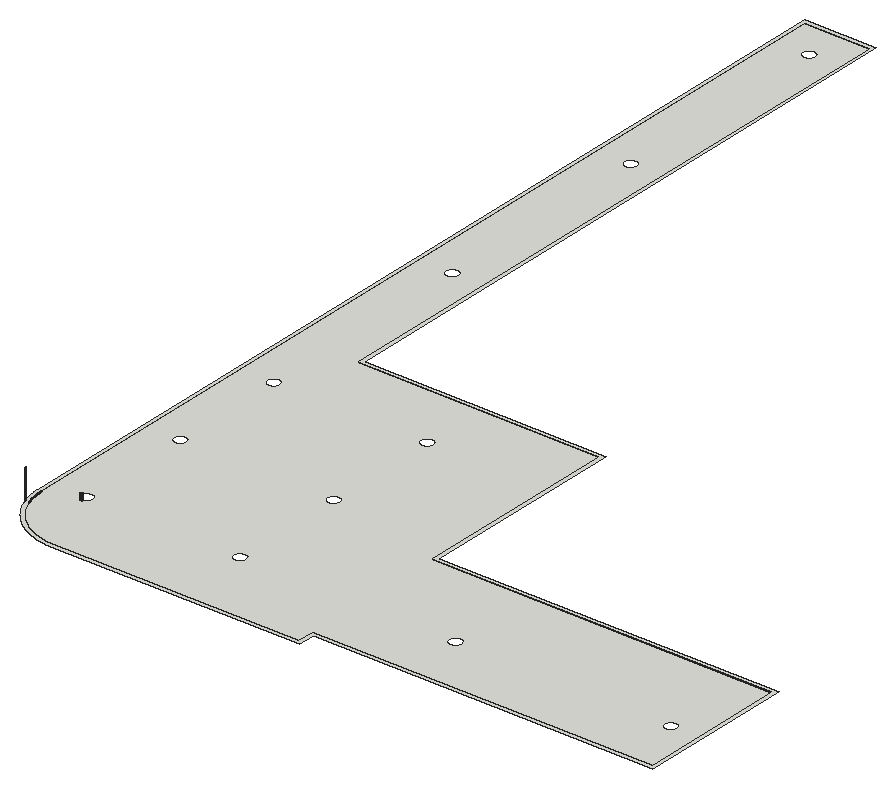
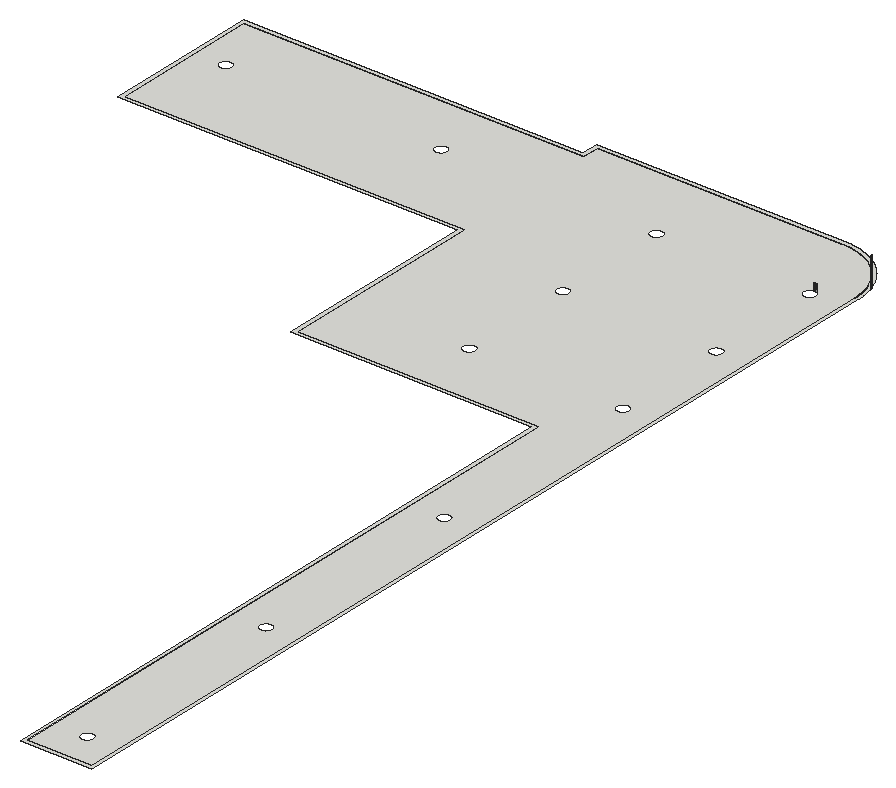
# SketchUp Ruby script. Lengths in inches.
U = 1.inch
M = Sketchup.active_model
def pt(a) = Geom::Point3d.new(a.map { |v| v * U })
def face(e, loops, mat)
  f = e.add_face(loops[0].map { |a| pt(a) })
  loops[1..].each { |l| e.add_face(l.map { |a| pt(a) }).erase! }
  f.material = f.back_material = mat if mat
  f
end
# faces: each face lists its corners as indices into pts; further lists are holes
def faces(e, pts, list, mat = nil) = list.each { |f| face(e, (f[0].is_a?(Array) ? f : [f]).map { |l| l.map { |i| pts[i] } }, mat) }
# xy, xz, yz: faces in a plane at the given z, y or x. An outline is a flat list of corners, or four numbers for a rectangle; further outlines are holes
def ring(l) = l.size == 4 ? [[l[0], l[1]], [l[2], l[1]], [l[2], l[3]], [l[0], l[3]]] : l.each_slice(2).to_a
def flat(e, list, mat, &to3) = list.each { |f| face(e, (f[0].is_a?(Array) ? f : [f]).map { |l| ring(l).map { |u, v| to3.(u, v) } }, mat) }
def xy(e, z, list, mat = nil) = flat(e, list, mat) { |x, y| [x, y, z] }
def xz(e, y, list, mat = nil) = flat(e, list, mat) { |x, z| [x, y, z] }
def yz(e, x, list, mat = nil) = flat(e, list, mat) { |y, z| [x, y, z] }
def lines(e, pts, list) = list.each { |a, b| e.add_line(pt(pts[a]), pt(pts[b])) }
# prism: a flat outline (further loops are holes) pulled along v
def prism(e, loops, v, mat = nil)
  f = face(e, loops, mat); d = Geom::Vector3d.new(v.map { |x| x * U })
  f.pushpull(f.normal.samedirection?(d) ? d.length : -d.length)
end
def box(e, o, s, mat = nil) = prism(e, [[o, [o[0] + s[0], o[1], o[2]], [o[0] + s[0], o[1] + s[1], o[2]], [o[0], o[1] + s[1], o[2]]]], [0, 0, s[2]], mat)
def at(x, y, z, deg = 0) = Geom::Transformation.translation(pt([x, y, z])) * Geom::Transformation.rotation(ORIGIN, Z_AXIS, deg.degrees)
def axes(o, x, y, z) = Geom::Transformation.new([*x, 0, *y, 0, *z, 0, *pt(o).to_a, 1])
def part(name) = M.definitions.add(name)
# library, detail: a bought-in or finely detailed component or shape, given as its bounding box
def library(name, o, s) = part(name).tap { |d| box(d.entities, o, s) }
def detail(e, o, s) = box(e.add_group.entities, o, s)
def put(e, d, t, mat = nil) = e.add_instance(d, t).tap { |i| i.material = mat if mat }
def group(e, t, mat = nil) = e.add_group.tap { |g| g.transformation = t; g.material = mat if mat }.entities
root = M.entities
M.materials.add("1496 AP 8293 CARBON COPY").color = [58, 58, 58]
xy(root,129,[[[43.625,86.5,43.25,86.51,42.88,86.52,42.51,86.54,42.14,86.5625,41.76,86.59,41.39,86.62,40.28,86.74,39.91,86.79,39.17,86.91,38.81,86.98,38.07,87.12,37.71,87.2,37.35,87.29,36.98,87.375,36.625,87.47,36.26,87.57,35.91,87.67,35.19,87.89,34.49,88.13,33.79,88.39,33.4375,88.53,33.09,88.67,32.75,88.8125,32.41,88.96,31.73,89.28,31.39,89.4375,31.0625,89.61,30.73,89.78,30.4,89.95,30.07,90.13,29.11,90.7,28.79,90.9,28.17,91.3,27.86,91.51,27.55,91.73,27.25,91.94,26.95,92.16,26.65,92.39,26.36,92.62,26.0625,92.85,25.78,93.09,25.49,93.33,25.21,93.57,24.65,94.07,24.11,94.59,23.59,95.11,23.07,95.65,22.57,96.21,22.33,96.49,22.09,96.78,21.85,97.0625,21.62,97.36,21.39,97.65,21.16,97.95,20.94,98.25,20.73,98.55,20.51,98.86,20.3,99.17,19.9,99.79,19.7,100.11,19.13,101.07,18.95,101.4,18.78,101.73,18.61,102.0625,18.4375,102.39,18.28,102.73,17.96,103.41,17.8125,103.75,17.67,104.09,17.53,104.4375,17.39,104.79,17.13,105.49,16.89,106.19,16.67,106.91,16.57,107.26,16.47,107.625,16.375,107.98,16.29,108.35,16.2,108.71,16.12,109.07,15.98,109.81,15.91,110.17,15.79,110.91,15.74,111.28,15.62,112.39,15.59,112.76,15.5625,113.14,15.54,113.51,15.52,113.88,15.51,114.25,15.5,114.625,15.5,553.5,45.5,553.5,45.5,259.5,156.5,259.5,156.5,163.5,312.5,163.5,312.5,94.5,156.5,94.5,156.5,86.5],[30.34,534,30.66,534,30.74,534.01,30.8125,534.02,30.89,534.03,31.05,534.05,31.125,534.07,31.2,534.08,31.28,534.1,31.35,534.125,31.43,534.15,31.5,534.17,31.58,534.2,31.79,534.29,31.86,534.33,31.93,534.36,32.07,534.44,32.13,534.48,32.2,534.53,32.26,534.57,32.33,534.62,32.57,534.82,32.62,534.88,32.68,534.93,32.88,535.17,32.93,535.24,32.97,535.3,33.02,535.37,33.06,535.43,33.14,535.57,33.17,535.64,33.21,535.71,33.3,535.92,33.33,536,33.35,536.07,33.375,536.15,33.4,536.22,33.42,536.3,33.43,536.375,33.45,536.45,33.47,536.61,33.48,536.6875,33.49,536.76,33.5,536.84,33.5,537.16,33.49,537.24,33.48,537.3125,33.47,537.39,33.45,537.55,33.43,537.625,33.42,537.7,33.4,537.78,33.375,537.85,33.35,537.93,33.33,538,33.3,538.08,33.21,538.29,33.17,538.36,33.14,538.43,33.06,538.57,33.02,538.63,32.97,538.7,32.93,538.76,32.88,538.83,32.68,539.07,32.62,539.12,32.57,539.18,32.33,539.38,32.26,539.43,32.2,539.47,32.13,539.52,32.07,539.56,31.93,539.64,31.86,539.67,31.79,539.71,31.58,539.8,31.5,539.83,31.43,539.85,31.35,539.875,31.28,539.9,31.2,539.92,31.125,539.93,31.05,539.95,30.89,539.97,30.8125,539.98,30.74,539.99,30.66,540,30.34,540,30.26,539.99,30.1875,539.98,30.11,539.97,29.95,539.95,29.875,539.93,29.8,539.92,29.72,539.9,29.65,539.875,29.57,539.85,29.5,539.83,29.42,539.8,29.21,539.71,29.14,539.67,29.07,539.64,28.93,539.56,28.87,539.52,28.8,539.47,28.74,539.43,28.67,539.38,28.43,539.18,28.38,539.12,28.32,539.07,28.12,538.83,28.07,538.76,28.03,538.7,27.98,538.63,27.94,538.57,27.86,538.43,27.83,538.36,27.79,538.29,27.7,538.08,27.67,538,27.65,537.93,27.625,537.85,27.6,537.78,27.58,537.7,27.57,537.625,27.55,537.55,27.53,537.39,27.52,537.3125,27.51,537.24,27.5,537.16,27.5,536.84,27.51,536.76,27.52,536.6875,27.53,536.61,27.55,536.45,27.57,536.375,27.58,536.3,27.6,536.22,27.625,536.15,27.65,536.07,27.67,536,27.7,535.92,27.79,535.71,27.83,535.64,27.86,535.57,27.94,535.43,27.98,535.37,28.03,535.3,28.07,535.24,28.12,535.17,28.32,534.93,28.38,534.88,28.43,534.82,28.67,534.62,28.74,534.57,28.8,534.53,28.87,534.48,28.93,534.44,29.07,534.36,29.14,534.33,29.21,534.29,29.42,534.2,29.5,534.17,29.57,534.15,29.65,534.125,29.72,534.1,29.8,534.08,29.875,534.07,29.95,534.05,30.11,534.03,30.1875,534.02,30.26,534.01],[30.34,329,30.66,329,30.74,329.01,30.8125,329.02,30.89,329.03,31.05,329.05,31.125,329.07,31.2,329.08,31.28,329.1,31.35,329.125,31.43,329.15,31.5,329.17,31.58,329.2,31.79,329.29,31.86,329.33,31.93,329.36,32.07,329.44,32.13,329.48,32.2,329.53,32.26,329.57,32.33,329.62,32.57,329.82,32.62,329.88,32.68,329.93,32.88,330.17,32.93,330.24,32.97,330.3,33.02,330.37,33.06,330.43,33.14,330.57,33.17,330.64,33.21,330.71,33.3,330.92,33.33,331,33.35,331.07,33.375,331.15,33.4,331.22,33.42,331.3,33.43,331.375,33.45,331.45,33.47,331.61,33.48,331.6875,33.49,331.76,33.5,331.84,33.5,332.16,33.49,332.24,33.48,332.3125,33.47,332.39,33.45,332.55,33.43,332.625,33.42,332.7,33.4,332.78,33.375,332.85,33.35,332.93,33.33,333,33.3,333.08,33.21,333.29,33.17,333.36,33.14,333.43,33.06,333.57,33.02,333.63,32.97,333.7,32.93,333.76,32.88,333.83,32.68,334.07,32.62,334.12,32.57,334.18,32.33,334.38,32.26,334.43,32.2,334.47,32.13,334.52,32.07,334.56,31.93,334.64,31.86,334.67,31.79,334.71,31.58,334.8,31.5,334.83,31.43,334.85,31.35,334.875,31.28,334.9,31.2,334.92,31.125,334.93,31.05,334.95,30.89,334.97,30.8125,334.98,30.74,334.99,30.66,335,30.34,335,30.26,334.99,30.1875,334.98,30.11,334.97,29.95,334.95,29.875,334.93,29.8,334.92,29.72,334.9,29.65,334.875,29.57,334.85,29.5,334.83,29.42,334.8,29.21,334.71,29.14,334.67,29.07,334.64,28.93,334.56,28.87,334.52,28.8,334.47,28.74,334.43,28.67,334.38,28.43,334.18,28.38,334.12,28.32,334.07,28.12,333.83,28.07,333.76,28.03,333.7,27.98,333.63,27.94,333.57,27.86,333.43,27.83,333.36,27.79,333.29,27.7,333.08,27.67,333,27.65,332.93,27.625,332.85,27.6,332.78,27.58,332.7,27.57,332.625,27.55,332.55,27.53,332.39,27.52,332.3125,27.51,332.24,27.5,332.16,27.5,331.84,27.51,331.76,27.52,331.6875,27.53,331.61,27.55,331.45,27.57,331.375,27.58,331.3,27.6,331.22,27.625,331.15,27.65,331.07,27.67,331,27.7,330.92,27.79,330.71,27.83,330.64,27.86,330.57,27.94,330.43,27.98,330.37,28.03,330.3,28.07,330.24,28.12,330.17,28.32,329.93,28.38,329.88,28.43,329.82,28.67,329.62,28.74,329.57,28.8,329.53,28.87,329.48,28.93,329.44,29.07,329.36,29.14,329.33,29.21,329.29,29.42,329.2,29.5,329.17,29.57,329.15,29.65,329.125,29.72,329.1,29.8,329.08,29.875,329.07,29.95,329.05,30.11,329.03,30.1875,329.02,30.26,329.01],[30.34,431.5,30.66,431.5,30.74,431.51,30.8125,431.52,30.89,431.53,31.05,431.55,31.125,431.57,31.2,431.58,31.28,431.6,31.35,431.625,31.43,431.65,31.5,431.67,31.58,431.7,31.79,431.79,31.86,431.83,31.93,431.86,32.07,431.94,32.13,431.98,32.2,432.03,32.26,432.07,32.33,432.12,32.57,432.32,32.62,432.38,32.68,432.43,32.88,432.67,32.93,432.74,32.97,432.8,33.02,432.87,33.06,432.93,33.14,433.07,33.17,433.14,33.21,433.21,33.3,433.42,33.33,433.5,33.35,433.57,33.375,433.65,33.4,433.72,33.42,433.8,33.43,433.875,33.45,433.95,33.47,434.11,33.48,434.1875,33.49,434.26,33.5,434.34,33.5,434.66,33.49,434.74,33.48,434.8125,33.47,434.89,33.45,435.05,33.43,435.125,33.42,435.2,33.4,435.28,33.375,435.35,33.35,435.43,33.33,435.5,33.3,435.58,33.21,435.79,33.17,435.86,33.14,435.93,33.06,436.07,33.02,436.13,32.97,436.2,32.93,436.26,32.88,436.33,32.68,436.57,32.62,436.62,32.57,436.68,32.33,436.88,32.26,436.93,32.2,436.97,32.13,437.02,32.07,437.06,31.93,437.14,31.86,437.17,31.79,437.21,31.58,437.3,31.5,437.33,31.43,437.35,31.35,437.375,31.28,437.4,31.2,437.42,31.125,437.43,31.05,437.45,30.89,437.47,30.8125,437.48,30.74,437.49,30.66,437.5,30.34,437.5,30.26,437.49,30.1875,437.48,30.11,437.47,29.95,437.45,29.875,437.43,29.8,437.42,29.72,437.4,29.65,437.375,29.57,437.35,29.5,437.33,29.42,437.3,29.21,437.21,29.14,437.17,29.07,437.14,28.93,437.06,28.87,437.02,28.8,436.97,28.74,436.93,28.67,436.88,28.43,436.68,28.38,436.62,28.32,436.57,28.12,436.33,28.07,436.26,28.03,436.2,27.98,436.13,27.94,436.07,27.86,435.93,27.83,435.86,27.79,435.79,27.7,435.58,27.67,435.5,27.65,435.43,27.625,435.35,27.6,435.28,27.58,435.2,27.57,435.125,27.55,435.05,27.53,434.89,27.52,434.8125,27.51,434.74,27.5,434.66,27.5,434.34,27.51,434.26,27.52,434.1875,27.53,434.11,27.55,433.95,27.57,433.875,27.58,433.8,27.6,433.72,27.625,433.65,27.65,433.57,27.67,433.5,27.7,433.42,27.79,433.21,27.83,433.14,27.86,433.07,27.94,432.93,27.98,432.87,28.03,432.8,28.07,432.74,28.12,432.67,28.32,432.43,28.38,432.38,28.43,432.32,28.67,432.12,28.74,432.07,28.8,432.03,28.87,431.98,28.93,431.94,29.07,431.86,29.14,431.83,29.21,431.79,29.42,431.7,29.5,431.67,29.57,431.65,29.65,431.625,29.72,431.6,29.8,431.58,29.875,431.57,29.95,431.55,30.11,431.53,30.1875,431.52,30.26,431.51],[100.84,226.5,101.16,226.5,101.24,226.51,101.3125,226.52,101.39,226.53,101.55,226.55,101.625,226.57,101.7,226.58,101.78,226.6,101.85,226.625,101.93,226.65,102,226.67,102.08,226.7,102.29,226.79,102.36,226.83,102.43,226.86,102.57,226.94,102.63,226.98,102.7,227.03,102.76,227.07,102.83,227.12,103.07,227.32,103.12,227.38,103.18,227.43,103.38,227.67,103.43,227.74,103.47,227.8,103.52,227.87,103.56,227.93,103.64,228.07,103.67,228.14,103.71,228.21,103.8,228.42,103.83,228.5,103.85,228.57,103.875,228.65,103.9,228.72,103.92,228.8,103.93,228.875,103.95,228.95,103.97,229.11,103.98,229.1875,103.99,229.26,104,229.34,104,229.66,103.99,229.74,103.98,229.8125,103.97,229.89,103.95,230.05,103.93,230.125,103.92,230.2,103.9,230.28,103.875,230.35,103.85,230.43,103.83,230.5,103.8,230.58,103.71,230.79,103.67,230.86,103.64,230.93,103.56,231.07,103.52,231.13,103.47,231.2,103.43,231.26,103.38,231.33,103.18,231.57,103.12,231.62,103.07,231.68,102.83,231.88,102.76,231.93,102.7,231.97,102.63,232.02,102.57,232.06,102.43,232.14,102.36,232.17,102.29,232.21,102.08,232.3,102,232.33,101.93,232.35,101.85,232.375,101.78,232.4,101.7,232.42,101.625,232.43,101.55,232.45,101.39,232.47,101.3125,232.48,101.24,232.49,101.16,232.5,100.84,232.5,100.76,232.49,100.6875,232.48,100.61,232.47,100.45,232.45,100.375,232.43,100.3,232.42,100.22,232.4,100.15,232.375,100.07,232.35,100,232.33,99.92,232.3,99.71,232.21,99.64,232.17,99.57,232.14,99.43,232.06,99.37,232.02,99.3,231.97,99.24,231.93,99.17,231.88,98.93,231.68,98.88,231.62,98.82,231.57,98.62,231.33,98.57,231.26,98.53,231.2,98.48,231.13,98.44,231.07,98.36,230.93,98.33,230.86,98.29,230.79,98.2,230.58,98.17,230.5,98.15,230.43,98.125,230.35,98.1,230.28,98.08,230.2,98.07,230.125,98.05,230.05,98.03,229.89,98.02,229.8125,98.01,229.74,98,229.66,98,229.34,98.01,229.26,98.02,229.1875,98.03,229.11,98.05,228.95,98.07,228.875,98.08,228.8,98.1,228.72,98.125,228.65,98.15,228.57,98.17,228.5,98.2,228.42,98.29,228.21,98.33,228.14,98.36,228.07,98.44,227.93,98.48,227.87,98.53,227.8,98.57,227.74,98.62,227.67,98.82,227.43,98.88,227.38,98.93,227.32,99.17,227.12,99.24,227.07,99.3,227.03,99.37,226.98,99.43,226.94,99.57,226.86,99.64,226.83,99.71,226.79,99.92,226.7,100,226.67,100.07,226.65,100.15,226.625,100.22,226.6,100.3,226.58,100.375,226.57,100.45,226.55,100.61,226.53,100.6875,226.52,100.76,226.51],[30.34,226.5,30.66,226.5,30.74,226.51,30.8125,226.52,30.89,226.53,31.05,226.55,31.125,226.57,31.2,226.58,31.28,226.6,31.35,226.625,31.43,226.65,31.5,226.67,31.58,226.7,31.79,226.79,31.86,226.83,31.93,226.86,32.07,226.94,32.13,226.98,32.2,227.03,32.26,227.07,32.33,227.12,32.57,227.32,32.62,227.38,32.68,227.43,32.88,227.67,32.93,227.74,32.97,227.8,33.02,227.87,33.06,227.93,33.14,228.07,33.17,228.14,33.21,228.21,33.3,228.42,33.33,228.5,33.35,228.57,33.375,228.65,33.4,228.72,33.42,228.8,33.43,228.875,33.45,228.95,33.47,229.11,33.48,229.1875,33.49,229.26,33.5,229.34,33.5,229.66,33.49,229.74,33.48,229.8125,33.47,229.89,33.45,230.05,33.43,230.125,33.42,230.2,33.4,230.28,33.375,230.35,33.35,230.43,33.33,230.5,33.3,230.58,33.21,230.79,33.17,230.86,33.14,230.93,33.06,231.07,33.02,231.13,32.97,231.2,32.93,231.26,32.88,231.33,32.68,231.57,32.62,231.62,32.57,231.68,32.33,231.88,32.26,231.93,32.2,231.97,32.13,232.02,32.07,232.06,31.93,232.14,31.86,232.17,31.79,232.21,31.58,232.3,31.5,232.33,31.43,232.35,31.35,232.375,31.28,232.4,31.2,232.42,31.125,232.43,31.05,232.45,30.89,232.47,30.8125,232.48,30.74,232.49,30.66,232.5,30.34,232.5,30.26,232.49,30.1875,232.48,30.11,232.47,29.95,232.45,29.875,232.43,29.8,232.42,29.72,232.4,29.65,232.375,29.57,232.35,29.5,232.33,29.42,232.3,29.21,232.21,29.14,232.17,29.07,232.14,28.93,232.06,28.87,232.02,28.8,231.97,28.74,231.93,28.67,231.88,28.43,231.68,28.38,231.62,28.32,231.57,28.12,231.33,28.07,231.26,28.03,231.2,27.98,231.13,27.94,231.07,27.86,230.93,27.83,230.86,27.79,230.79,27.7,230.58,27.67,230.5,27.65,230.43,27.625,230.35,27.6,230.28,27.58,230.2,27.57,230.125,27.55,230.05,27.53,229.89,27.52,229.8125,27.51,229.74,27.5,229.66,27.5,229.34,27.51,229.26,27.52,229.1875,27.53,229.11,27.55,228.95,27.57,228.875,27.58,228.8,27.6,228.72,27.625,228.65,27.65,228.57,27.67,228.5,27.7,228.42,27.79,228.21,27.83,228.14,27.86,228.07,27.94,227.93,27.98,227.87,28.03,227.8,28.07,227.74,28.12,227.67,28.32,227.43,28.38,227.38,28.43,227.32,28.67,227.12,28.74,227.07,28.8,227.03,28.87,226.98,28.93,226.94,29.07,226.86,29.14,226.83,29.21,226.79,29.42,226.7,29.5,226.67,29.57,226.65,29.65,226.625,29.72,226.6,29.8,226.58,29.875,226.57,29.95,226.55,30.11,226.53,30.1875,226.52,30.26,226.51],[100.84,172.75,101.16,172.75,101.24,172.76,101.3125,172.77,101.39,172.78,101.55,172.8,101.625,172.82,101.7,172.83,101.78,172.85,101.85,172.875,101.93,172.9,102,172.92,102.08,172.95,102.29,173.04,102.36,173.08,102.43,173.11,102.57,173.19,102.63,173.23,102.7,173.28,102.76,173.32,102.83,173.37,103.07,173.57,103.12,173.63,103.18,173.68,103.38,173.92,103.43,173.99,103.47,174.05,103.52,174.12,103.56,174.18,103.64,174.32,103.67,174.39,103.71,174.46,103.8,174.67,103.83,174.75,103.85,174.82,103.875,174.9,103.9,174.97,103.92,175.05,103.93,175.125,103.95,175.2,103.97,175.36,103.98,175.4375,103.99,175.51,104,175.59,104,175.91,103.99,175.99,103.98,176.0625,103.97,176.14,103.95,176.3,103.93,176.375,103.92,176.45,103.9,176.53,103.875,176.6,103.85,176.68,103.83,176.75,103.8,176.83,103.71,177.04,103.67,177.11,103.64,177.18,103.56,177.32,103.52,177.38,103.47,177.45,103.43,177.51,103.38,177.58,103.18,177.82,103.12,177.87,103.07,177.93,102.83,178.13,102.76,178.18,102.7,178.22,102.63,178.27,102.57,178.31,102.43,178.39,102.36,178.42,102.29,178.46,102.08,178.55,102,178.58,101.93,178.6,101.85,178.625,101.78,178.65,101.7,178.67,101.625,178.68,101.55,178.7,101.39,178.72,101.3125,178.73,101.24,178.74,101.16,178.75,100.84,178.75,100.76,178.74,100.6875,178.73,100.61,178.72,100.45,178.7,100.375,178.68,100.3,178.67,100.22,178.65,100.15,178.625,100.07,178.6,100,178.58,99.92,178.55,99.71,178.46,99.64,178.42,99.57,178.39,99.43,178.31,99.37,178.27,99.3,178.22,99.24,178.18,99.17,178.13,98.93,177.93,98.88,177.87,98.82,177.82,98.62,177.58,98.57,177.51,98.53,177.45,98.48,177.38,98.44,177.32,98.36,177.18,98.33,177.11,98.29,177.04,98.2,176.83,98.17,176.75,98.15,176.68,98.125,176.6,98.1,176.53,98.08,176.45,98.07,176.375,98.05,176.3,98.03,176.14,98.02,176.0625,98.01,175.99,98,175.91,98,175.59,98.01,175.51,98.02,175.4375,98.03,175.36,98.05,175.2,98.07,175.125,98.08,175.05,98.1,174.97,98.125,174.9,98.15,174.82,98.17,174.75,98.2,174.67,98.29,174.46,98.33,174.39,98.36,174.32,98.44,174.18,98.48,174.12,98.53,174.05,98.57,173.99,98.62,173.92,98.82,173.68,98.88,173.63,98.93,173.57,99.17,173.37,99.24,173.32,99.3,173.28,99.37,173.23,99.43,173.19,99.57,173.11,99.64,173.08,99.71,173.04,99.92,172.95,100,172.92,100.07,172.9,100.15,172.875,100.22,172.85,100.3,172.83,100.375,172.82,100.45,172.8,100.61,172.78,100.6875,172.77,100.76,172.76],[100.84,119,101.16,119,101.24,119.01,101.3125,119.02,101.39,119.03,101.55,119.05,101.625,119.07,101.7,119.08,101.78,119.1,101.85,119.125,101.93,119.15,102,119.17,102.08,119.2,102.29,119.29,102.36,119.33,102.43,119.36,102.57,119.44,102.63,119.48,102.7,119.53,102.76,119.57,102.83,119.62,103.07,119.82,103.12,119.88,103.18,119.93,103.38,120.17,103.43,120.24,103.47,120.3,103.52,120.37,103.56,120.43,103.64,120.57,103.67,120.64,103.71,120.71,103.8,120.92,103.83,121,103.85,121.07,103.875,121.15,103.9,121.22,103.92,121.3,103.93,121.375,103.95,121.45,103.97,121.61,103.98,121.6875,103.99,121.76,104,121.84,104,122.16,103.99,122.24,103.98,122.3125,103.97,122.39,103.95,122.55,103.93,122.625,103.92,122.7,103.9,122.78,103.875,122.85,103.85,122.93,103.83,123,103.8,123.08,103.71,123.29,103.67,123.36,103.64,123.43,103.56,123.57,103.52,123.63,103.47,123.7,103.43,123.76,103.38,123.83,103.18,124.07,103.12,124.12,103.07,124.18,102.83,124.38,102.76,124.43,102.7,124.47,102.63,124.52,102.57,124.56,102.43,124.64,102.36,124.67,102.29,124.71,102.08,124.8,102,124.83,101.93,124.85,101.85,124.875,101.78,124.9,101.7,124.92,101.625,124.93,101.55,124.95,101.39,124.97,101.3125,124.98,101.24,124.99,101.16,125,100.84,125,100.76,124.99,100.6875,124.98,100.61,124.97,100.45,124.95,100.375,124.93,100.3,124.92,100.22,124.9,100.15,124.875,100.07,124.85,100,124.83,99.92,124.8,99.71,124.71,99.64,124.67,99.57,124.64,99.43,124.56,99.37,124.52,99.3,124.47,99.24,124.43,99.17,124.38,98.93,124.18,98.88,124.12,98.82,124.07,98.62,123.83,98.57,123.76,98.53,123.7,98.48,123.63,98.44,123.57,98.36,123.43,98.33,123.36,98.29,123.29,98.2,123.08,98.17,123,98.15,122.93,98.125,122.85,98.1,122.78,98.08,122.7,98.07,122.625,98.05,122.55,98.03,122.39,98.02,122.3125,98.01,122.24,98,122.16,98,121.84,98.01,121.76,98.02,121.6875,98.03,121.61,98.05,121.45,98.07,121.375,98.08,121.3,98.1,121.22,98.125,121.15,98.15,121.07,98.17,121,98.2,120.92,98.29,120.71,98.33,120.64,98.36,120.57,98.44,120.43,98.48,120.37,98.53,120.3,98.57,120.24,98.62,120.17,98.82,119.93,98.88,119.88,98.93,119.82,99.17,119.62,99.24,119.57,99.3,119.53,99.37,119.48,99.43,119.44,99.57,119.36,99.64,119.33,99.71,119.29,99.92,119.2,100,119.17,100.07,119.15,100.15,119.125,100.22,119.1,100.3,119.08,100.375,119.07,100.45,119.05,100.61,119.03,100.6875,119.02,100.76,119.01],[199.84,119,200.16,119,200.24,119.01,200.3125,119.02,200.39,119.03,200.55,119.05,200.625,119.07,200.7,119.08,200.78,119.1,200.85,119.125,200.93,119.15,201,119.17,201.08,119.2,201.29,119.29,201.36,119.33,201.43,119.36,201.57,119.44,201.63,119.48,201.7,119.53,201.76,119.57,201.83,119.62,202.07,119.82,202.12,119.88,202.18,119.93,202.38,120.17,202.43,120.24,202.47,120.3,202.52,120.37,202.56,120.43,202.64,120.57,202.67,120.64,202.71,120.71,202.8,120.92,202.83,121,202.85,121.07,202.875,121.15,202.9,121.22,202.92,121.3,202.93,121.375,202.95,121.45,202.97,121.61,202.98,121.6875,202.99,121.76,203,121.84,203,122.16,202.99,122.24,202.98,122.3125,202.97,122.39,202.95,122.55,202.93,122.625,202.92,122.7,202.9,122.78,202.875,122.85,202.85,122.93,202.83,123,202.8,123.08,202.71,123.29,202.67,123.36,202.64,123.43,202.56,123.57,202.52,123.63,202.47,123.7,202.43,123.76,202.38,123.83,202.18,124.07,202.12,124.12,202.07,124.18,201.83,124.38,201.76,124.43,201.7,124.47,201.63,124.52,201.57,124.56,201.43,124.64,201.36,124.67,201.29,124.71,201.08,124.8,201,124.83,200.93,124.85,200.85,124.875,200.78,124.9,200.7,124.92,200.625,124.93,200.55,124.95,200.39,124.97,200.3125,124.98,200.24,124.99,200.16,125,199.84,125,199.76,124.99,199.6875,124.98,199.61,124.97,199.45,124.95,199.375,124.93,199.3,124.92,199.22,124.9,199.15,124.875,199.07,124.85,199,124.83,198.92,124.8,198.71,124.71,198.64,124.67,198.57,124.64,198.43,124.56,198.37,124.52,198.3,124.47,198.24,124.43,198.17,124.38,197.93,124.18,197.88,124.12,197.82,124.07,197.62,123.83,197.57,123.76,197.53,123.7,197.48,123.63,197.44,123.57,197.36,123.43,197.33,123.36,197.29,123.29,197.2,123.08,197.17,123,197.15,122.93,197.125,122.85,197.1,122.78,197.08,122.7,197.07,122.625,197.05,122.55,197.03,122.39,197.02,122.3125,197.01,122.24,197,122.16,197,121.84,197.01,121.76,197.02,121.6875,197.03,121.61,197.05,121.45,197.07,121.375,197.08,121.3,197.1,121.22,197.125,121.15,197.15,121.07,197.17,121,197.2,120.92,197.29,120.71,197.33,120.64,197.36,120.57,197.44,120.43,197.48,120.37,197.53,120.3,197.57,120.24,197.62,120.17,197.82,119.93,197.88,119.88,197.93,119.82,198.17,119.62,198.24,119.57,198.3,119.53,198.37,119.48,198.43,119.44,198.57,119.36,198.64,119.33,198.71,119.29,198.92,119.2,199,119.17,199.07,119.15,199.15,119.125,199.22,119.1,199.3,119.08,199.375,119.07,199.45,119.05,199.61,119.03,199.6875,119.02,199.76,119.01],[298.84,119,299.16,119,299.24,119.01,299.3125,119.02,299.39,119.03,299.55,119.05,299.625,119.07,299.7,119.08,299.78,119.1,299.85,119.125,299.93,119.15,300,119.17,300.08,119.2,300.29,119.29,300.36,119.33,300.43,119.36,300.57,119.44,300.63,119.48,300.7,119.53,300.76,119.57,300.83,119.62,301.07,119.82,301.12,119.88,301.18,119.93,301.38,120.17,301.43,120.24,301.47,120.3,301.52,120.37,301.56,120.43,301.64,120.57,301.67,120.64,301.71,120.71,301.8,120.92,301.83,121,301.85,121.07,301.875,121.15,301.9,121.22,301.92,121.3,301.93,121.375,301.95,121.45,301.97,121.61,301.98,121.6875,301.99,121.76,302,121.84,302,122.16,301.99,122.24,301.98,122.3125,301.97,122.39,301.95,122.55,301.93,122.625,301.92,122.7,301.9,122.78,301.875,122.85,301.85,122.93,301.83,123,301.8,123.08,301.71,123.29,301.67,123.36,301.64,123.43,301.56,123.57,301.52,123.63,301.47,123.7,301.43,123.76,301.38,123.83,301.18,124.07,301.12,124.12,301.07,124.18,300.83,124.38,300.76,124.43,300.7,124.47,300.63,124.52,300.57,124.56,300.43,124.64,300.36,124.67,300.29,124.71,300.08,124.8,300,124.83,299.93,124.85,299.85,124.875,299.78,124.9,299.7,124.92,299.625,124.93,299.55,124.95,299.39,124.97,299.3125,124.98,299.24,124.99,299.16,125,298.84,125,298.76,124.99,298.6875,124.98,298.61,124.97,298.45,124.95,298.375,124.93,298.3,124.92,298.22,124.9,298.15,124.875,298.07,124.85,298,124.83,297.92,124.8,297.71,124.71,297.64,124.67,297.57,124.64,297.43,124.56,297.37,124.52,297.3,124.47,297.24,124.43,297.17,124.38,296.93,124.18,296.88,124.12,296.82,124.07,296.62,123.83,296.57,123.76,296.53,123.7,296.48,123.63,296.44,123.57,296.36,123.43,296.33,123.36,296.29,123.29,296.2,123.08,296.17,123,296.15,122.93,296.125,122.85,296.1,122.78,296.08,122.7,296.07,122.625,296.05,122.55,296.03,122.39,296.02,122.3125,296.01,122.24,296,122.16,296,121.84,296.01,121.76,296.02,121.6875,296.03,121.61,296.05,121.45,296.07,121.375,296.08,121.3,296.1,121.22,296.125,121.15,296.15,121.07,296.17,121,296.2,120.92,296.29,120.71,296.33,120.64,296.36,120.57,296.44,120.43,296.48,120.37,296.53,120.3,296.57,120.24,296.62,120.17,296.82,119.93,296.88,119.88,296.93,119.82,297.17,119.62,297.24,119.57,297.3,119.53,297.37,119.48,297.43,119.44,297.57,119.36,297.64,119.33,297.71,119.29,297.92,119.2,298,119.17,298.07,119.15,298.15,119.125,298.22,119.1,298.3,119.08,298.375,119.07,298.45,119.05,298.61,119.03,298.6875,119.02,298.76,119.01],[30.34,172.75,30.66,172.75,30.74,172.76,30.8125,172.77,30.89,172.78,31.05,172.8,31.125,172.82,31.2,172.83,31.28,172.85,31.35,172.875,31.43,172.9,31.5,172.92,31.58,172.95,31.79,173.04,31.86,173.08,31.93,173.11,32.07,173.19,32.13,173.23,32.2,173.28,32.26,173.32,32.33,173.37,32.57,173.57,32.62,173.63,32.68,173.68,32.88,173.92,32.93,173.99,32.97,174.05,33.02,174.12,33.06,174.18,33.14,174.32,33.17,174.39,33.21,174.46,33.3,174.67,33.33,174.75,33.35,174.82,33.375,174.9,33.4,174.97,33.42,175.05,33.43,175.125,33.45,175.2,33.47,175.36,33.48,175.4375,33.49,175.51,33.5,175.59,33.5,175.91,33.49,175.99,33.48,176.0625,33.47,176.14,33.45,176.3,33.43,176.375,33.42,176.45,33.4,176.53,33.375,176.6,33.35,176.68,33.33,176.75,33.3,176.83,33.21,177.04,33.17,177.11,33.14,177.18,33.06,177.32,33.02,177.38,32.97,177.45,32.93,177.51,32.88,177.58,32.68,177.82,32.62,177.87,32.57,177.93,32.33,178.13,32.26,178.18,32.2,178.22,32.13,178.27,32.07,178.31,31.93,178.39,31.86,178.42,31.79,178.46,31.58,178.55,31.5,178.58,31.43,178.6,31.35,178.625,31.28,178.65,31.2,178.67,31.125,178.68,31.05,178.7,30.89,178.72,30.8125,178.73,30.74,178.74,30.66,178.75,30.34,178.75,30.26,178.74,30.1875,178.73,30.11,178.72,29.95,178.7,29.875,178.68,29.8,178.67,29.72,178.65,29.65,178.625,29.57,178.6,29.5,178.58,29.42,178.55,29.21,178.46,29.14,178.42,29.07,178.39,28.93,178.31,28.87,178.27,28.8,178.22,28.74,178.18,28.67,178.13,28.43,177.93,28.38,177.87,28.32,177.82,28.12,177.58,28.07,177.51,28.03,177.45,27.98,177.38,27.94,177.32,27.86,177.18,27.83,177.11,27.79,177.04,27.7,176.83,27.67,176.75,27.65,176.68,27.625,176.6,27.6,176.53,27.58,176.45,27.57,176.375,27.55,176.3,27.53,176.14,27.52,176.0625,27.51,175.99,27.5,175.91,27.5,175.59,27.51,175.51,27.52,175.4375,27.53,175.36,27.55,175.2,27.57,175.125,27.58,175.05,27.6,174.97,27.625,174.9,27.65,174.82,27.67,174.75,27.7,174.67,27.79,174.46,27.83,174.39,27.86,174.32,27.94,174.18,27.98,174.12,28.03,174.05,28.07,173.99,28.12,173.92,28.32,173.68,28.38,173.63,28.43,173.57,28.67,173.37,28.74,173.32,28.8,173.28,28.87,173.23,28.93,173.19,29.07,173.11,29.14,173.08,29.21,173.04,29.42,172.95,29.5,172.92,29.57,172.9,29.65,172.875,29.72,172.85,29.8,172.83,29.875,172.82,29.95,172.8,30.11,172.78,30.1875,172.77,30.26,172.76],[30.34,119,30.66,119,30.74,119.01,30.8125,119.02,30.89,119.03,31.05,119.05,31.125,119.07,31.2,119.08,31.28,119.1,31.35,119.125,31.43,119.15,31.5,119.17,31.58,119.2,31.79,119.29,31.86,119.33,31.93,119.36,32.07,119.44,32.13,119.48,32.2,119.53,32.26,119.57,32.33,119.62,32.57,119.82,32.62,119.88,32.68,119.93,32.88,120.17,32.93,120.24,32.97,120.3,33.02,120.37,33.06,120.43,33.14,120.57,33.17,120.64,33.21,120.71,33.3,120.92,33.33,121,33.35,121.07,33.375,121.15,33.4,121.22,33.42,121.3,33.43,121.375,33.45,121.45,33.47,121.61,33.48,121.6875,33.49,121.76,33.5,121.84,33.5,122.16,33.49,122.24,33.48,122.3125,33.47,122.39,33.45,122.55,33.43,122.625,33.42,122.7,33.4,122.78,33.375,122.85,33.35,122.93,33.33,123,33.3,123.08,33.21,123.29,33.17,123.36,33.14,123.43,33.06,123.57,33.02,123.63,32.97,123.7,32.93,123.76,32.88,123.83,32.68,124.07,32.62,124.12,32.57,124.18,32.33,124.38,32.26,124.43,32.2,124.47,32.13,124.52,32.07,124.56,31.93,124.64,31.86,124.67,31.79,124.71,31.58,124.8,31.5,124.83,31.43,124.85,31.35,124.875,31.28,124.9,31.2,124.92,31.125,124.93,31.05,124.95,30.89,124.97,30.8125,124.98,30.74,124.99,30.66,125,30.34,125,30.26,124.99,30.1875,124.98,30.11,124.97,29.95,124.95,29.875,124.93,29.8,124.92,29.72,124.9,29.65,124.875,29.57,124.85,29.5,124.83,29.42,124.8,29.21,124.71,29.14,124.67,29.07,124.64,28.93,124.56,28.87,124.52,28.8,124.47,28.74,124.43,28.67,124.38,28.43,124.18,28.38,124.12,28.32,124.07,28.12,123.83,28.07,123.76,28.03,123.7,27.98,123.63,27.94,123.57,27.86,123.43,27.83,123.36,27.79,123.29,27.7,123.08,27.67,123,27.65,122.93,27.625,122.85,27.6,122.78,27.58,122.7,27.57,122.625,27.55,122.55,27.53,122.39,27.52,122.3125,27.51,122.24,27.5,122.16,27.5,121.84,27.51,121.76,27.52,121.6875,27.53,121.61,27.55,121.45,27.57,121.375,27.58,121.3,27.6,121.22,27.625,121.15,27.65,121.07,27.67,121,27.7,120.92,27.79,120.71,27.83,120.64,27.86,120.57,27.94,120.43,27.98,120.37,28.03,120.3,28.07,120.24,28.12,120.17,28.32,119.93,28.38,119.88,28.43,119.82,28.67,119.62,28.74,119.57,28.8,119.53,28.87,119.48,28.93,119.44,29.07,119.36,29.14,119.33,29.21,119.29,29.42,119.2,29.5,119.17,29.57,119.15,29.65,119.125,29.72,119.1,29.8,119.08,29.875,119.07,29.95,119.05,30.11,119.03,30.1875,119.02,30.26,119.01]]])
xy(root,129.5,[[[43.61,85,43.21,85.01,42.82,85.02,42.43,85.04,42.04,85.0625,41.65,85.09,41.25,85.125,40.86,85.16,40.08,85.26,39.7,85.31,38.92,85.43,38.53,85.5,38.15,85.58,37.76,85.66,37.38,85.74,36.62,85.92,36.24,86.02,35.86,86.125,35.48,86.24,35.1,86.35,34.36,86.59,33.62,86.85,33.25,86.99,32.88,87.14,32.52,87.28,32.16,87.4375,31.8,87.59,31.44,87.76,31.08,87.92,30.73,88.09,30.03,88.45,29.69,88.64,29.34,88.83,29,89.02,28.66,89.22,28.33,89.42,27.99,89.63,27.66,89.84,27.33,90.06,27.01,90.28,26.6875,90.5,26.37,90.73,26.05,90.96,25.43,91.44,25.12,91.6875,24.82,91.93,24.52,92.1875,24.22,92.44,23.93,92.71,23.64,92.97,23.35,93.24,23.07,93.51,22.51,94.07,22.24,94.35,21.97,94.64,21.71,94.93,21.44,95.22,21.1875,95.52,20.93,95.82,20.6875,96.12,20.44,96.43,19.96,97.05,19.73,97.37,19.5,97.6875,19.28,98.01,19.06,98.33,18.84,98.66,18.63,98.99,18.42,99.33,18.22,99.66,18.02,100,17.83,100.34,17.64,100.69,17.45,101.03,17.09,101.73,16.92,102.08,16.76,102.44,16.59,102.8,16.4375,103.16,16.28,103.52,16.14,103.88,15.99,104.25,15.85,104.62,15.59,105.36,15.35,106.1,15.24,106.48,15.125,106.86,15.02,107.24,14.92,107.62,14.74,108.38,14.66,108.76,14.58,109.15,14.5,109.53,14.43,109.92,14.31,110.7,14.26,111.08,14.16,111.86,14.125,112.25,14.09,112.65,14.0625,113.04,14.04,113.43,14.02,113.82,14.01,114.21,14,114.61,14,555,47,555,47,261,158,261,158,165,314,165,314,93,158,93,158,85],[43.625,86.5,156.5,86.5,156.5,94.5,312.5,94.5,312.5,163.5,156.5,163.5,156.5,259.5,45.5,259.5,45.5,553.5,15.5,553.5,15.5,114.625,15.51,114.25,15.52,113.88,15.54,113.51,15.5625,113.14,15.59,112.76,15.62,112.39,15.74,111.28,15.79,110.91,15.91,110.17,15.98,109.81,16.12,109.07,16.2,108.71,16.29,108.35,16.375,107.98,16.47,107.625,16.57,107.26,16.67,106.91,16.89,106.19,17.13,105.49,17.39,104.79,17.53,104.4375,17.67,104.09,17.8125,103.75,17.96,103.41,18.28,102.73,18.4375,102.39,18.61,102.0625,18.78,101.73,18.95,101.4,19.13,101.07,19.7,100.11,19.9,99.79,20.3,99.17,20.51,98.86,20.73,98.55,20.94,98.25,21.16,97.95,21.39,97.65,21.62,97.36,21.85,97.0625,22.09,96.78,22.33,96.49,22.57,96.21,23.07,95.65,23.59,95.11,24.11,94.59,24.65,94.07,25.21,93.57,25.49,93.33,25.78,93.09,26.0625,92.85,26.36,92.62,26.65,92.39,26.95,92.16,27.25,91.94,27.55,91.73,27.86,91.51,28.17,91.3,28.79,90.9,29.11,90.7,30.07,90.13,30.4,89.95,30.73,89.78,31.0625,89.61,31.39,89.4375,31.73,89.28,32.41,88.96,32.75,88.8125,33.09,88.67,33.4375,88.53,33.79,88.39,34.49,88.13,35.19,87.89,35.91,87.67,36.26,87.57,36.625,87.47,36.98,87.375,37.35,87.29,37.71,87.2,38.07,87.12,38.81,86.98,39.17,86.91,39.91,86.79,40.28,86.74,41.39,86.62,41.76,86.59,42.14,86.5625,42.51,86.54,42.88,86.52,43.25,86.51]]])
xz(root,119,[[30.34,129,30.42,132],[30.42,129,30.5,132],[30.5,129,30.58,132],[30.58,129,30.66,132]])
yz(root,15.5,[[114.625,129,115,129.5]])
p = [[15.72,104.99,129],[15.59,105.36,129],[15.59,105.36,143],[15.72,104.99,143],[17.13,105.49,129],[17.26,105.14,129],
  [17.26,105.14,129.5],[17.13,105.49,129.5],[15.47,105.73,129],[15.47,105.73,143],[17.01,105.84,129],[17.01,105.84,129.5],
  [15.35,106.1,129],[15.35,106.1,143],[16.89,106.19,129],[16.89,106.19,129.5],[16.78,106.55,129],[16.78,106.55,129.5],
  [16.67,106.91,129],[16.67,106.91,129.5],[16.57,107.26,129],[16.57,107.26,129.5],[16.47,107.625,129],[16.47,107.625,129.5],
  [16.375,107.98,129],[16.375,107.98,129.5],[16.29,108.35,129],[16.29,108.35,129.5],[16.2,108.71,129],[16.2,108.71,129.5],
  [16.12,109.07,129],[16.12,109.07,129.5],[16.05,109.44,129],[16.05,109.44,129.5],[15.98,109.81,129],[15.98,109.81,129.5],
  [15.91,110.17,129],[15.91,110.17,129.5],[15.85,110.54,129],[15.85,110.54,129.5],[15.79,110.91,129],[15.79,110.91,129.5],
  [15.74,111.28,129],[15.74,111.28,129.5],[15.7,111.65,129],[15.7,111.65,129.5],[15.66,112.02,129],[15.66,112.02,129.5],
  [15.62,112.39,129],[15.62,112.39,129.5],[15.59,112.76,129],[15.59,112.76,129.5],[15.5625,113.14,129],[15.5625,113.14,129.5],
  [15.54,113.51,129],[15.54,113.51,129.5],[15.52,113.88,129],[15.52,113.88,129.5],[15.51,114.25,129],[15.51,114.25,129.5],
  [15.5,114.625,129],[15.5,114.625,129.5],[30.03,119.04,129],[29.95,119.05,129],[29.95,119.05,132],[30.03,119.04,132],
  [30.11,119.03,129],[30.11,119.03,132],[30.1875,119.02,129],[30.1875,119.02,132],[30.26,119.01,129],[30.26,119.01,132],
  [30.34,119,129],[30.34,119,132],[30.74,119.01,129],[30.66,119,129],[30.66,119,132],[30.74,119.01,132],
  [30.8125,119.02,129],[30.8125,119.02,132],[30.89,119.03,129],[30.89,119.03,132],[30.97,119.04,129],[30.97,119.04,132],
  [31.05,119.05,129],[31.05,119.05,132],[29.875,119.07,129],[29.875,119.07,132],[15.59,105.36,138],[15.47,105.73,138],
  [15.47,105.73,129.5],[15.59,105.36,129.5]]
faces(root,p,[[0,1,2,3],[1,8,9,2],[8,12,13,9]],"1496 AP 8293 CARBON COPY")
faces(root,p,[[4,5,6,7],[10,4,7,11],[14,10,11,15],[16,14,15,17],[18,16,17,19],[20,18,19,21],[22,20,21,23],[24,22,23,25],
  [26,24,25,27],[28,26,27,29],[30,28,29,31],[32,30,31,33],[34,32,33,35],[36,34,35,37],[38,36,37,39],[40,38,39,41],
  [42,40,41,43],[44,42,43,45],[46,44,45,47],[48,46,47,49],[50,48,49,51],[52,50,51,53],[54,52,53,55],[56,54,55,57],
  [58,56,57,59],[60,58,59,61],[62,63,64,65],[66,62,65,67],[68,66,67,69],[70,68,69,71],[72,70,71,73],[74,75,76,77],
  [78,74,77,79],[80,78,79,81],[82,80,81,83],[84,82,83,85],[63,86,87,64],[88,89,90,91]])
